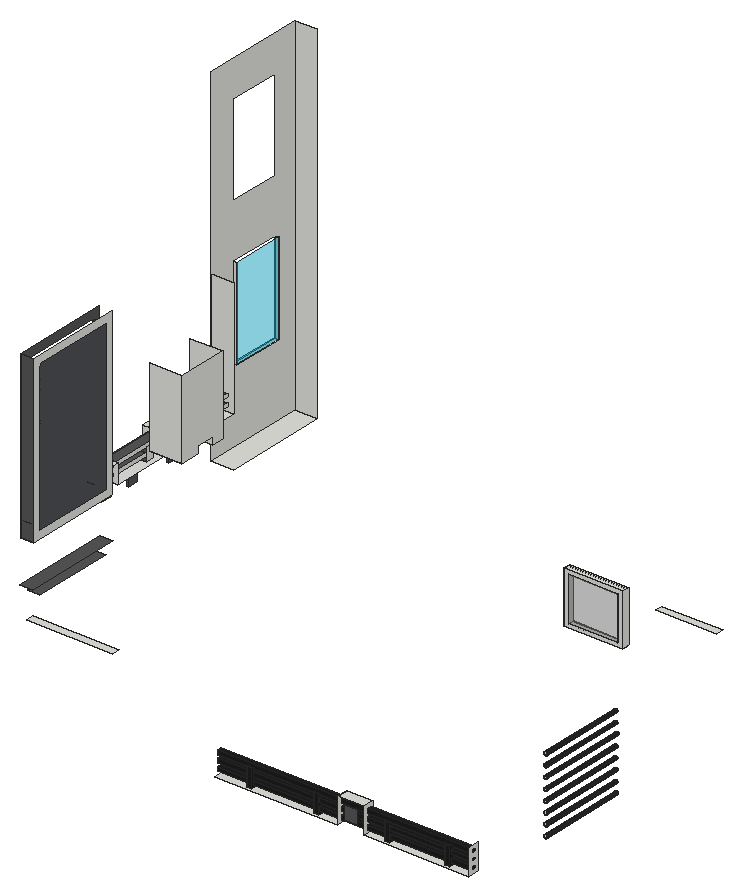
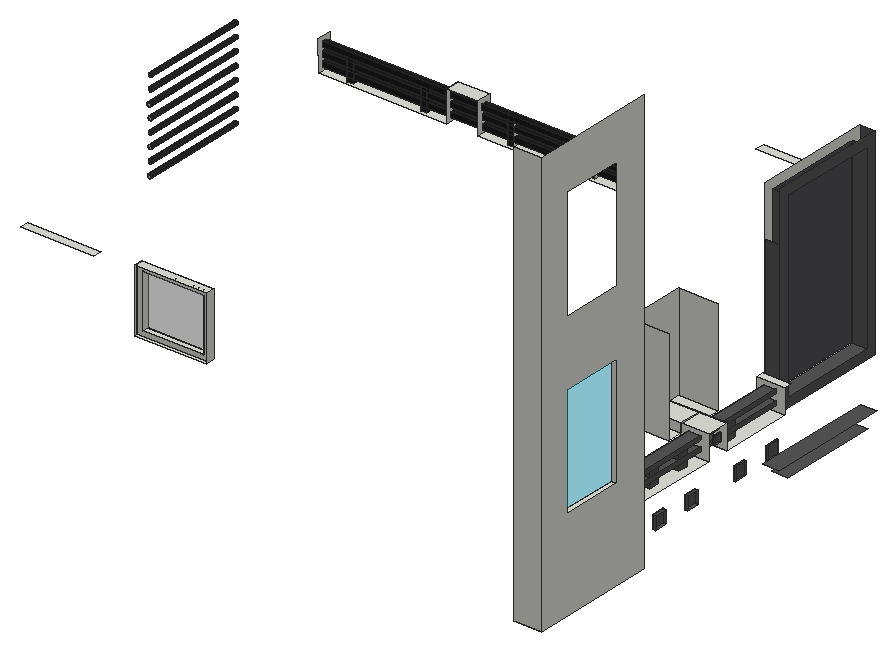
# SketchUp Ruby script. Lengths in inches.
U = 1.inch
M = Sketchup.active_model
def pt(a) = Geom::Point3d.new(a.map { |v| v * U })
def face(e, loops, mat)
  f = e.add_face(loops[0].map { |a| pt(a) })
  loops[1..].each { |l| e.add_face(l.map { |a| pt(a) }).erase! }
  f.material = f.back_material = mat if mat
  f
end
# faces: each face lists its corners as indices into pts; further lists are holes
def faces(e, pts, list, mat = nil) = list.each { |f| face(e, (f[0].is_a?(Array) ? f : [f]).map { |l| l.map { |i| pts[i] } }, mat) }
# xy, xz, yz: faces in a plane at the given z, y or x. An outline is a flat list of corners, or four numbers for a rectangle; further outlines are holes
def ring(l) = l.size == 4 ? [[l[0], l[1]], [l[2], l[1]], [l[2], l[3]], [l[0], l[3]]] : l.each_slice(2).to_a
def flat(e, list, mat, &to3) = list.each { |f| face(e, (f[0].is_a?(Array) ? f : [f]).map { |l| ring(l).map { |u, v| to3.(u, v) } }, mat) }
def xy(e, z, list, mat = nil) = flat(e, list, mat) { |x, y| [x, y, z] }
def xz(e, y, list, mat = nil) = flat(e, list, mat) { |x, z| [x, y, z] }
def yz(e, x, list, mat = nil) = flat(e, list, mat) { |y, z| [x, y, z] }
def lines(e, pts, list) = list.each { |a, b| e.add_line(pt(pts[a]), pt(pts[b])) }
# prism: a flat outline (further loops are holes) pulled along v
def prism(e, loops, v, mat = nil)
  f = face(e, loops, mat); d = Geom::Vector3d.new(v.map { |x| x * U })
  f.pushpull(f.normal.samedirection?(d) ? d.length : -d.length)
end
def box(e, o, s, mat = nil) = prism(e, [[o, [o[0] + s[0], o[1], o[2]], [o[0] + s[0], o[1] + s[1], o[2]], [o[0], o[1] + s[1], o[2]]]], [0, 0, s[2]], mat)
def at(x, y, z, deg = 0) = Geom::Transformation.translation(pt([x, y, z])) * Geom::Transformation.rotation(ORIGIN, Z_AXIS, deg.degrees)
def axes(o, x, y, z) = Geom::Transformation.new([*x, 0, *y, 0, *z, 0, *pt(o).to_a, 1])
def part(name) = M.definitions.add(name)
# library, detail: a bought-in or finely detailed component or shape, given as its bounding box
def library(name, o, s) = part(name).tap { |d| box(d.entities, o, s) }
def detail(e, o, s) = box(e.add_group.entities, o, s)
def put(e, d, t, mat = nil) = e.add_instance(d, t).tap { |i| i.material = mat if mat }
def group(e, t, mat = nil) = e.add_group.tap { |g| g.transformation = t; g.material = mat if mat }.entities
root = M.entities
M.materials.add("[Blinds Roman Hobbled Blue]").color = [81, 82, 87]
M.materials.add("[Color M06]").color = [86, 86, 86]
M.materials.add("[Color M08]").color = [30, 30, 30]
M.materials.add("[Translucent Glass Gray]").color = [128, 128, 128]
M.materials["[Translucent Glass Gray]"].alpha = 0.5
M.materials.add("[Translucent Glass Tinted]").color = [8, 201, 241]
M.materials["[Translucent Glass Tinted]"].alpha = 0.48
c1 = part("Group\#4")
xy(c1.entities,0,[[0,0,32.875,4]])
xy(c1.entities,2.47,[[2.47,0,30.4,4]])
xy(c1.entities,30.4,[[2.47,0,30.4,4]])
xy(c1.entities,32.875,[[0,0,32.875,4]])
xz(c1.entities,0,[[[0,0,32.875,32.875],[2.47,2.47,30.4,30.4]]])
xz(c1.entities,0,[[2.47,2.47,30.4,30.4]],"[Translucent Glass Gray]")
xz(c1.entities,4,[[[0,0,32.875,32.875],[2.47,2.47,30.4,30.4]]])
yz(c1.entities,0,[[0,0,4,32.875]])
yz(c1.entities,2.47,[[0,2.47,4,30.4]])
yz(c1.entities,30.4,[[0,2.47,4,30.4]])
yz(c1.entities,32.875,[[0,0,4,32.875]])
xy(root,185.33,[[67.1875,170.55,77.4375,235.42]],"[Color M06]")
xy(root,189.3125,[[[310.75,52.875,408.29,62.01],[387.07,55.5,391.07,59.5],[333.89,55.5,337.89,59.5]],[[428.93,52.875,512.75,62.01],[491.95,55.5,495.95,59.5],[443.64,55.5,447.64,59.5]]])
xy(root,190.375,[[59.3125,362.77,77.4375,446.27]])
xy(root,191.91,[[310.75,56.1,512.75,59.54]])
xy(root,192.66,[[67.1875,163.22,77.4375,242.75]],"[Color M06]")
xy(root,192.97,[[364.5,332.8125,411.32,338.8125]])
xy(root,195.34,[[310.75,56.1,512.75,59.54]],"[Color M08]")
xy(root,197.91,[[310.125,56.1,512.75,59.54]])
xy(root,201.34,[[310.125,56.1,512.75,59.54]],"[Color M08]")
xy(root,203.72,[[310.25,56.2,310.25,59.64,512.75,59.64,512.75,56.2,447.64,56.2,447.64,59.5,443.64,59.5,443.64,56.2],[443.64,56.2,447.64,59.5]])
xy(root,203.72,[[443.64,55.5,447.64,56.2]],"[Color M08]")
xy(root,204.125,[[333.89,55.5,337.89,59.5],[491.95,55.5,495.95,59.5]],"[Color M08]")
xy(root,204.5,[[387.07,55.5,391.07,59.5]],"[Color M08]")
xy(root,207.16,[[310.25,56.2,512.75,59.64]],"[Color M08]")
xy(root,208.79,[[59.3125,279.625,60.5,288.1875],[59.3125,318.6875,61.375,327.25],[59.3125,344.8125,61.3125,353.375]],"[Color M06]")
xy(root,209.47,[[59.3125,253.3125,60.3125,261.875]],"[Color M06]")
xy(root,209.8125,[[408.29,52.875,428.93,62.01]])
xy(root,217.35,[[59.3125,279.625,60.5,288.1875],[59.3125,318.6875,61.375,327.25],[59.3125,344.8125,61.3125,353.375]],"[Color M06]")
xy(root,218.03,[[59.3125,253.3125,60.3125,261.875]],"[Color M06]")
xy(root,225.6875,[[67.1875,164.28,77.4375,241.6875]],"[Color M06]")
xy(root,230,[[438.18,332.8125,486.18,338.8125]])
xy(root,231.95,[[67.1875,170.55,77.4375,235.42]],"[Color M06]")
xy(root,233.875,[[64.69,248.07,72.82,365.76]],"[Color M06]")
xy(root,234.22,[[364.5,332.8125,411.32,338.8125]])
xy(root,236.6875,[[64.69,248.07,72.82,365.76]],"[Color M06]")
xy(root,237.48,[[59.3125,300.15,60.1875,305.34]],"[Color M06]")
xy(root,240.34,[[77.4375,279.8125,103.125,294.97],[77.4375,309.77,103.125,319.875]])
xy(root,240.5,[[64.69,248.07,72.82,367.07]],"[Color M06]")
xy(root,242.66,[[59.3125,300.15,60.1875,305.34]],"[Color M06]")
xy(root,243.3125,[[64.69,248.07,72.82,367.07]],"[Color M06]")
xy(root,245.87,[[157.85,56.875,226.03,62.875]])
xy(root,246.02,[[59.3125,242.75,77.4375,248.07],[59.3125,294.97,77.4375,309.77],[77.4375,294.97,103.125,309.77]])
xy(root,250.33,[[59.3125,385.09,62.5,426.22]])
xz(root,52.875,[[414.09,194.96,423.78,205.53]],"[Color M06]")
xz(root,55.5,[[333.89,189.3125,337.89,204.125],[387.07,189.3125,391.07,204.5],[443.64,189.3125,447.64,203.72],[491.95,189.3125,495.95,204.125]],"[Color M08]")
xz(root,56.1,[[310.75,191.91,512.75,195.34],[310.125,197.91,512.75,201.34]],"[Color M08]")
xz(root,56.2,[[310.25,203.72,512.75,207.16]],"[Color M08]")
xz(root,59.5,[[333.89,189.3125,337.89,204.125],[387.07,189.3125,391.07,204.5],[443.64,189.3125,447.64,203.72],[491.95,189.3125,495.95,204.125]],"[Color M08]")
xz(root,59.54,[[310.75,191.91,512.75,195.34],[310.125,197.91,512.75,201.34]],"[Color M08]")
xz(root,59.64,[[310.25,203.72,512.75,207.16]],"[Color M08]")
xz(root,125.55,[[515.8,185.63,516.12,185.67,516.42,185.8,516.68,186,516.88,186.26,517.01,186.56,517.05,186.88,517.01,187.2,516.88,187.51,516.68,187.76,516.42,187.96,516.12,188.09,515.8,188.13,515.47,188.09,515.17,187.96,514.91,187.76,514.72,187.51,514.59,187.2,514.55,186.88,514.59,186.56,514.72,186.26,514.91,186,515.17,185.8,515.47,185.67],[515.8,194.07,516.12,194.11,516.42,194.24,516.68,194.43,516.88,194.69,517.01,194.99,517.05,195.32,517.01,195.64,516.88,195.94,516.68,196.2,516.42,196.4,516.12,196.53,515.8,196.57,515.47,196.53,515.17,196.4,514.91,196.2,514.72,195.94,514.59,195.64,514.55,195.32,514.59,194.99,514.72,194.69,514.91,194.43,515.17,194.24,515.47,194.11],[515.8,202.51,516.12,202.55,516.42,202.67,516.68,202.87,516.88,203.13,517.01,203.43,517.05,203.76,517.01,204.08,516.88,204.38,516.68,204.64,516.42,204.84,516.12,204.96,515.8,205.01,515.47,204.96,515.17,204.84,514.91,204.64,514.72,204.38,514.59,204.08,514.55,203.76,514.59,203.43,514.72,203.13,514.91,202.87,515.17,202.67,515.47,202.55],[515.8,210.94,516.12,210.99,516.42,211.11,516.68,211.31,516.88,211.57,517.01,211.87,517.05,212.19,517.01,212.52,516.88,212.82,516.68,213.08,516.42,213.28,516.12,213.4,515.8,213.44,515.47,213.4,515.17,213.28,514.91,213.08,514.72,212.82,514.59,212.52,514.55,212.19,514.59,211.87,514.72,211.57,514.91,211.31,515.17,211.11,515.47,210.99],[515.8,219.38,516.12,219.42,516.42,219.55,516.68,219.75,516.88,220.01,517.01,220.31,517.05,220.63,517.01,220.95,516.88,221.26,516.68,221.51,516.42,221.71,516.12,221.84,515.8,221.88,515.47,221.84,515.17,221.71,514.91,221.51,514.72,221.26,514.59,220.95,514.55,220.63,514.59,220.31,514.72,220.01,514.91,219.75,515.17,219.55,515.47,219.42],
  [515.8,227.82,516.12,227.86,516.42,227.99,516.68,228.18,516.88,228.44,517.01,228.74,517.05,229.07,517.01,229.39,516.88,229.69,516.68,229.95,516.42,230.15,516.12,230.28,515.8,230.32,515.47,230.28,515.17,230.15,514.91,229.95,514.72,229.69,514.59,229.39,514.55,229.07,514.59,228.74,514.72,228.44,514.91,228.18,515.17,227.99,515.47,227.86],[515.8,244.69,516.12,244.74,516.42,244.86,516.68,245.06,516.88,245.32,517.01,245.62,517.05,245.94,517.01,246.27,516.88,246.57,516.68,246.83,516.42,247.03,516.12,247.15,515.8,247.19,515.47,247.15,515.17,247.03,514.91,246.83,514.72,246.57,514.59,246.27,514.55,245.94,514.59,245.62,514.72,245.32,514.91,245.06,515.17,244.86,515.47,244.74]])
xz(root,164.28,[[67.1875,225.6875,77.4375,356.84]],"[Color M06]")
xz(root,170.55,[[67.1875,231.95,77.4375,350.58]],"[Color M06]")
xz(root,195.68,[[515.8,219.38,515.47,219.42,515.17,219.55,514.91,219.75,514.72,220.01,514.59,220.31,514.55,220.63,514.59,220.95,514.72,221.26,514.91,221.51,515.17,221.71,515.47,221.84,515.8,221.88,516.12,221.84,516.42,221.71,516.68,221.51,516.88,221.26,517.01,220.95,517.05,220.63,517.01,220.31,516.88,220.01,516.68,219.75,516.42,219.55,516.12,219.42]])
xz(root,195.74,[[515.8,202.51,515.47,202.55,515.17,202.67,514.91,202.87,514.72,203.13,514.59,203.43,514.55,203.76,514.59,204.08,514.72,204.38,514.91,204.64,515.17,204.84,515.47,204.96,515.8,205.01,516.12,204.96,516.42,204.84,516.68,204.64,516.88,204.38,517.01,204.08,517.05,203.76,517.01,203.43,516.88,203.13,516.68,202.87,516.42,202.67,516.12,202.55]])
xz(root,196.24,[[515.8,185.63,515.47,185.67,515.17,185.8,514.91,186,514.72,186.26,514.59,186.56,514.55,186.88,514.59,187.2,514.72,187.51,514.91,187.76,515.17,187.96,515.47,188.09,515.8,188.13,516.12,188.09,516.42,187.96,516.68,187.76,516.88,187.51,517.01,187.2,517.05,186.88,517.01,186.56,516.88,186.26,516.68,186,516.42,185.8,516.12,185.67]])
xz(root,196.68,[[515.8,227.82,515.47,227.86,515.17,227.99,514.91,228.18,514.72,228.44,514.59,228.74,514.55,229.07,514.59,229.39,514.72,229.69,514.91,229.95,515.17,230.15,515.47,230.28,515.8,230.32,516.12,230.28,516.42,230.15,516.68,229.95,516.88,229.69,517.01,229.39,517.05,229.07,517.01,228.74,516.88,228.44,516.68,228.18,516.42,227.99,516.12,227.86]])
xz(root,235.42,[[67.1875,231.95,77.4375,350.58]],"[Color M06]")
xz(root,241.6875,[[67.1875,225.6875,77.4375,323.97]],"[Color M06]")
xz(root,248.07,[[[59.3125,230.24,77.4375,246.02],[64.69,233.875,72.82,236.6875],[64.69,240.5,72.82,243.3125]],[64.69,233.875,72.82,236.6875],[64.69,240.5,72.82,243.3125]])
xz(root,253.3125,[[59.3125,209.47,60.3125,218.03]],"[Color M06]")
xz(root,261.875,[[59.3125,209.47,60.3125,218.03]],"[Color M06]")
xz(root,279.625,[[59.3125,208.79,60.5,217.35]],"[Color M06]")
xz(root,279.8125,[[77.4375,240.34,103.125,302.91]])
xz(root,288.1875,[[59.3125,208.79,60.5,217.35]],"[Color M06]")
xz(root,294.97,[[59.3125,229.95,77.4375,246.02],[77.4375,240.34,103.125,246.02]])
xz(root,300.15,[[59.3125,237.48,60.1875,242.66]],"[Color M06]")
xz(root,305.34,[[59.3125,237.48,60.1875,242.66]],"[Color M06]")
xz(root,309.77,[[59.3125,229.95,77.4375,246.02],[77.4375,240.34,103.125,246.02]])
xz(root,318.6875,[[59.3125,208.79,61.375,217.35]],"[Color M06]")
xz(root,319.875,[[77.4375,240.34,103.125,302.91]])
xz(root,327.25,[[59.3125,208.79,61.375,217.35]],"[Color M06]")
xz(root,344.8125,[[59.3125,208.79,61.3125,217.35]],"[Color M06]")
xz(root,353.375,[[59.3125,208.79,61.3125,217.35]],"[Color M06]")
xz(root,362.77,[[59.3125,230.24,77.4375,323.97]])
xz(root,365.76,[[64.69,233.875,72.82,236.6875]])
xz(root,367.07,[[64.69,240.5,72.82,243.3125]])
xz(root,385.09,[[59.3125,250.33,62.5,323.27]])
xz(root,426.22,[[59.3125,250.33,62.5,323.27]])
xz(root,446.27,[[59.3125,190.375,77.4375,468]])
yz(root,59.3125,[[[362.77,190.375,446.27,468],[385.09,365.83,426.22,438.77],[385.09,250.33,426.22,323.27]]])
yz(root,60.1875,[[300.15,237.48,305.34,242.66]],"[Color M06]")
yz(root,60.3125,[[253.3125,209.47,261.875,218.03]],"[Color M06]")
yz(root,60.5,[[279.625,208.79,288.1875,217.35]],"[Color M06]")
yz(root,61.3125,[[344.8125,208.79,353.375,217.35]],"[Color M06]")
yz(root,61.375,[[318.6875,208.79,327.25,217.35]],"[Color M06]")
yz(root,62.5,[[385.09,250.33,426.22,323.27]],"[Translucent Glass Tinted]")
yz(root,64.69,[[248.07,233.875,365.76,236.6875],[248.07,240.5,367.07,243.3125]],"[Color M06]")
yz(root,64.87,[[281.6,230.14,281.54,241.27,287.67,241.3,287.73,230.17],[321.17,230.14,321.11,240.77,327.23,240.8,327.29,230.17],[344.73,230.14,344.67,240.5,350.8,240.54,350.85,230.17]],"[Color M06]")
yz(root,67.1875,[[[164.28,225.6875,241.6875,356.84],[170.55,231.95,235.42,350.58]]],"[Color M06]")
yz(root,72.82,[[248.07,233.875,365.76,236.6875],[248.07,240.5,367.07,243.3125]])
yz(root,73.43,[[281.6,230.14,287.73,230.17,287.67,241.3,281.54,241.27],[321.17,230.14,327.29,230.17,327.23,240.8,321.11,240.77],[344.73,230.14,350.85,230.17,350.8,240.54,344.67,240.5]])
yz(root,77.4375,[[[164.28,225.6875,241.6875,356.84],[170.55,231.95,235.42,350.58]],[294.97,240.34,309.77,246.02]])
yz(root,77.4375,[[170.55,231.95,235.42,350.58]],"[Blinds Roman Hobbled Blue]")
yz(root,103.125,[[279.8125,240.34,279.8125,302.91,319.875,302.91,319.875,240.34,309.77,240.34,309.77,246.02,294.97,246.02,294.97,240.34]])
yz(root,310.125,[[56.1,197.91,59.54,201.34]])
yz(root,310.25,[[56.2,203.72,59.64,207.16]])
yz(root,333.89,[[55.5,189.3125,59.5,204.125]])
yz(root,337.89,[[55.5,189.3125,59.5,204.125]],"[Color M08]")
yz(root,364.5,[[332.8125,192.97,338.8125,234.22]])
yz(root,387.07,[[55.5,189.3125,59.5,204.5]])
yz(root,391.07,[[55.5,189.3125,59.5,204.5]],"[Color M08]")
yz(root,408.29,[[52.875,189.3125,62.01,209.8125]])
yz(root,411.32,[[332.8125,192.97,338.8125,234.22]])
yz(root,428.93,[[52.875,189.3125,62.01,209.8125]])
yz(root,443.64,[[55.5,189.3125,59.5,203.72]],"[Color M08]")
yz(root,447.64,[[55.5,189.3125,59.5,203.72]],"[Color M08]")
yz(root,491.95,[[55.5,189.3125,59.5,204.125]],"[Color M08]")
yz(root,495.95,[[55.5,189.3125,59.5,204.125]],"[Color M08]")
yz(root,512.75,[[[52.875,189.3125,52.875,209.8125,62.375,209.8125,62.01,189.3125],[56.2,203.72,59.64,207.16],[56.1,197.91,59.54,201.34],[56.1,191.91,59.54,195.34]]])
p = [[515.8,125.55,185.63],[515.47,125.55,185.67],[515.47,196.24,185.67],[515.8,196.24,185.63],[516.12,125.55,185.67],[516.12,196.24,185.67],
  [515.17,125.55,185.8],[515.17,196.24,185.8],[516.42,125.55,185.8],[516.42,196.24,185.8],[514.91,125.55,186],[514.91,196.24,186],
  [516.68,125.55,186],[516.68,196.24,186],[514.72,125.55,186.26],[514.72,196.24,186.26],[516.88,125.55,186.26],[516.88,196.24,186.26],
  [514.59,125.55,186.56],[514.59,196.24,186.56],[517.01,125.55,186.56],[517.01,196.24,186.56],[514.55,125.55,186.88],[514.55,196.24,186.88],
  [517.05,125.55,186.88],[517.05,196.24,186.88],[514.59,125.55,187.2],[514.59,196.24,187.2],[517.01,125.55,187.2],[517.01,196.24,187.2],
  [514.72,125.55,187.51],[514.72,196.24,187.51],[516.88,125.55,187.51],[516.88,196.24,187.51],[514.91,125.55,187.76],[514.91,196.24,187.76],
  [516.68,125.55,187.76],[516.68,196.24,187.76],[515.17,125.55,187.96],[515.17,196.24,187.96],[516.42,125.55,187.96],[516.42,196.24,187.96],
  [515.47,125.55,188.09],[515.47,196.24,188.09],[516.12,125.55,188.09],[516.12,196.24,188.09],[515.8,125.55,188.13],[515.8,196.24,188.13],
  [515.47,125.55,194.11],[515.17,125.55,194.24],[515.17,195.62,194.24],[515.47,195.62,194.11],[515.8,125.55,194.07],[515.8,195.62,194.07],
  [516.12,125.55,194.11],[516.12,195.62,194.11],[516.42,125.55,194.24],[516.42,195.62,194.24],[514.91,125.55,194.43],[514.91,195.62,194.43],
  [516.68,125.55,194.43],[516.68,195.62,194.43],[514.72,125.55,194.69],[514.72,195.62,194.69],[516.88,125.55,194.69],[516.88,195.62,194.69],
  [514.59,125.55,194.99],[514.59,195.62,194.99],[517.01,125.55,194.99],[517.01,195.62,194.99],[514.55,125.55,195.32],[514.55,195.62,195.32],
  [517.05,125.55,195.32],[517.05,195.62,195.32],[514.59,125.55,195.64],[514.59,195.62,195.64],[517.01,125.55,195.64],[517.01,195.62,195.64],
  [514.72,125.55,195.94],[514.72,195.62,195.94],[516.88,125.55,195.94],[516.88,195.62,195.94],[514.91,125.55,196.2],[514.91,195.62,196.2],
  [516.68,125.55,196.2],[516.68,195.62,196.2],[515.17,125.55,196.4],[515.17,195.62,196.4],[516.42,125.55,196.4],[516.42,195.62,196.4],
  [515.47,125.55,196.53],[515.47,195.62,196.53],[516.12,125.55,196.53],[516.12,195.62,196.53],[515.8,125.55,196.57],[515.8,195.62,196.57],
  [515.47,125.55,202.55],[515.17,125.55,202.67],[515.17,195.74,202.67],[515.47,195.74,202.55],[515.8,125.55,202.51],[515.8,195.74,202.51],
  [516.12,125.55,202.55],[516.12,195.74,202.55],[516.42,125.55,202.67],[516.42,195.74,202.67],[514.91,125.55,202.87],[514.91,195.74,202.87],
  [516.68,125.55,202.87],[516.68,195.74,202.87],[514.72,125.55,203.13],[514.72,195.74,203.13],[516.88,125.55,203.13],[516.88,195.74,203.13],
  [514.59,125.55,203.43],[514.59,195.74,203.43],[517.01,125.55,203.43],[517.01,195.74,203.43],[514.55,125.55,203.76],[514.55,195.74,203.76],
  [517.05,125.55,203.76],[517.05,195.74,203.76],[514.59,125.55,204.08],[514.59,195.74,204.08],[517.01,125.55,204.08],[517.01,195.74,204.08],
  [514.72,125.55,204.38],[514.72,195.74,204.38],[516.88,125.55,204.38],[516.88,195.74,204.38],[514.91,125.55,204.64],[514.91,195.74,204.64],
  [516.68,125.55,204.64],[516.68,195.74,204.64],[515.17,125.55,204.84],[515.17,195.74,204.84],[516.42,125.55,204.84],[516.42,195.74,204.84],
  [515.47,125.55,204.96],[515.47,195.74,204.96],[516.12,125.55,204.96],[516.12,195.74,204.96],[515.8,125.55,205.01],[515.8,195.74,205.01],
  [515.8,125.55,210.94],[515.47,125.55,210.99],[515.47,195.62,210.99],[515.8,195.62,210.94],[516.12,125.55,210.99],[516.12,195.62,210.99],
  [515.17,125.55,211.11],[515.17,195.62,211.11],[516.42,125.55,211.11],[516.42,195.62,211.11],[514.91,125.55,211.31],[514.91,195.62,211.31],
  [516.68,125.55,211.31],[516.68,195.62,211.31],[514.72,125.55,211.57],[514.72,195.62,211.57],[516.88,125.55,211.57],[516.88,195.62,211.57],
  [514.59,125.55,211.87],[514.59,195.62,211.87],[517.01,125.55,211.87],[517.01,195.62,211.87],[514.55,125.55,212.19],[514.55,195.62,212.19],
  [517.05,125.55,212.19],[517.05,195.62,212.19],[514.59,125.55,212.52],[514.59,195.62,212.52],[517.01,125.55,212.52],[517.01,195.62,212.52],
  [514.72,125.55,212.82],[514.72,195.62,212.82],[516.88,125.55,212.82],[516.88,195.62,212.82],[514.91,125.55,213.08],[514.91,195.62,213.08],
  [516.68,125.55,213.08],[516.68,195.62,213.08],[515.17,125.55,213.28],[515.17,195.62,213.28],[516.42,125.55,213.28],[516.42,195.62,213.28],
  [515.47,125.55,213.4],[515.47,195.62,213.4],[516.12,125.55,213.4],[516.12,195.62,213.4],[515.8,125.55,213.44],[515.8,195.62,213.44],
  [515.47,125.55,219.42],[515.17,125.55,219.55],[515.17,195.68,219.55],[515.47,195.68,219.42],[515.8,125.55,219.38],[515.8,195.68,219.38],
  [516.12,125.55,219.42],[516.12,195.68,219.42],[516.42,125.55,219.55],[516.42,195.68,219.55],[514.91,125.55,219.75],[514.91,195.68,219.75],
  [516.68,125.55,219.75],[516.68,195.68,219.75],[514.72,125.55,220.01],[514.72,195.68,220.01],[516.88,125.55,220.01],[516.88,195.68,220.01],
  [514.59,125.55,220.31],[514.59,195.68,220.31],[517.01,125.55,220.31],[517.01,195.68,220.31],[514.55,125.55,220.63],[514.55,195.68,220.63],
  [517.05,125.55,220.63],[517.05,195.68,220.63],[514.59,125.55,220.95],[514.59,195.68,220.95],[517.01,125.55,220.95],[517.01,195.68,220.95],
  [514.72,125.55,221.26],[514.72,195.68,221.26],[516.88,125.55,221.26],[516.88,195.68,221.26],[514.91,125.55,221.51],[514.91,195.68,221.51],
  [516.68,125.55,221.51],[516.68,195.68,221.51],[515.17,125.55,221.71],[515.17,195.68,221.71],[516.42,125.55,221.71],[516.42,195.68,221.71],
  [515.47,125.55,221.84],[515.47,195.68,221.84],[516.12,125.55,221.84],[516.12,195.68,221.84],[515.8,125.55,221.88],[515.8,195.68,221.88],
  [515.8,125.55,227.82],[515.47,125.55,227.86],[515.47,196.68,227.86],[515.8,196.68,227.82],[516.12,125.55,227.86],[516.12,196.68,227.86],
  [515.17,125.55,227.99],[515.17,196.68,227.99],[516.42,125.55,227.99],[516.42,196.68,227.99],[514.91,125.55,228.18],[514.91,196.68,228.18],
  [516.68,125.55,228.18],[516.68,196.68,228.18],[514.72,125.55,228.44],[514.72,196.68,228.44],[516.88,125.55,228.44],[516.88,196.68,228.44],
  [514.59,125.55,228.74],[514.59,196.68,228.74],[517.01,125.55,228.74],[517.01,196.68,228.74],[514.55,125.55,229.07],[514.55,196.68,229.07],
  [517.05,125.55,229.07],[517.05,196.68,229.07],[514.59,125.55,229.39],[514.59,196.68,229.39],[517.01,125.55,229.39],[517.01,196.68,229.39],
  [514.72,125.55,229.69],[514.72,196.68,229.69],[516.88,125.55,229.69],[516.88,196.68,229.69],[514.91,125.55,229.95],[514.91,196.68,229.95],
  [516.68,125.55,229.95],[516.68,196.68,229.95],[515.17,125.55,230.15],[515.17,196.68,230.15],[516.42,125.55,230.15],[516.42,196.68,230.15],
  [77.4375,248.07,230.24],[77.4375,294.97,229.95],[59.3125,294.97,229.95],[59.3125,248.07,230.24],[59.3125,362.77,230.24],[59.3125,309.77,229.95],
  [77.4375,309.77,229.95],[77.4375,362.77,230.24],[73.43,344.73,230.14],[64.87,344.73,230.14],[64.87,350.85,230.17],[73.43,350.85,230.17],
  [64.87,281.6,230.14],[73.43,281.6,230.14],[73.43,281.54,241.27],[64.87,281.54,241.27],[64.87,287.73,230.17],[73.43,287.73,230.17],
  [64.87,321.17,230.14],[73.43,321.17,230.14],[73.43,321.11,240.77],[64.87,321.11,240.77],[64.87,327.29,230.17],[73.43,327.29,230.17],
  [73.43,344.67,240.5],[64.87,344.67,240.5],[515.47,125.55,230.28],[515.47,196.68,230.28],[516.12,125.55,230.28],[516.12,196.68,230.28],
  [64.87,287.67,241.3],[73.43,287.67,241.3],[64.87,327.23,240.8],[73.43,327.23,240.8],[64.87,350.8,240.54],[73.43,350.8,240.54],
  [515.8,125.55,230.32],[515.8,196.68,230.32],[515.47,125.55,236.3],[515.17,125.55,236.42],[515.17,195.62,236.42],[515.47,195.62,236.3],
  [515.8,125.55,236.26],[515.8,195.62,236.26],[516.12,125.55,236.3],[516.12,195.62,236.3],[516.42,125.55,236.42],[516.42,195.62,236.42],
  [514.91,125.55,236.62],[514.91,195.62,236.62],[516.68,125.55,236.62],[516.68,195.62,236.62],[514.72,125.55,236.88],[514.72,195.62,236.88],
  [516.88,125.55,236.88],[516.88,195.62,236.88],[514.59,125.55,237.18],[514.59,195.62,237.18],[517.01,125.55,237.18],[517.01,195.62,237.18],
  [514.55,125.55,237.51],[514.55,195.62,237.51],[517.05,125.55,237.51],[517.05,195.62,237.51],[514.59,125.55,237.83],[514.59,195.62,237.83],
  [517.01,125.55,237.83],[517.01,195.62,237.83],[514.72,125.55,238.13],[514.72,195.62,238.13],[516.88,125.55,238.13],[516.88,195.62,238.13],
  [514.91,125.55,238.39],[514.91,195.62,238.39],[516.68,125.55,238.39],[516.68,195.62,238.39],[515.17,125.55,238.59],[515.17,195.62,238.59],
  [516.42,125.55,238.59],[516.42,195.62,238.59],[515.47,125.55,238.71],[515.47,195.62,238.71],[516.12,125.55,238.71],[516.12,195.62,238.71],
  [515.8,125.55,238.76],[515.8,195.62,238.76],[515.47,125.55,244.74],[515.17,125.55,244.86],[515.17,195.62,244.86],[515.47,195.62,244.74],
  [515.8,125.55,244.69],[515.8,195.62,244.69],[516.12,125.55,244.74],[516.12,195.62,244.74],[516.42,125.55,244.86],[516.42,195.62,244.86],
  [514.91,125.55,245.06],[514.91,195.62,245.06],[516.68,125.55,245.06],[516.68,195.62,245.06],[514.72,125.55,245.32],[514.72,195.62,245.32],
  [516.88,125.55,245.32],[516.88,195.62,245.32],[514.59,125.55,245.62],[514.59,195.62,245.62],[517.01,125.55,245.62],[517.01,195.62,245.62],
  [514.55,125.55,245.94],[514.55,195.62,245.94],[517.05,125.55,245.94],[517.05,195.62,245.94],[514.59,125.55,246.27],[514.59,195.62,246.27],
  [517.01,125.55,246.27],[517.01,195.62,246.27],[514.72,125.55,246.57],[514.72,195.62,246.57],[516.88,125.55,246.57],[516.88,195.62,246.57],
  [514.91,125.55,246.83],[514.91,195.62,246.83],[516.68,125.55,246.83],[516.68,195.62,246.83],[515.17,125.55,247.03],[515.17,195.62,247.03],
  [516.42,125.55,247.03],[516.42,195.62,247.03],[515.47,125.55,247.15],[515.47,195.62,247.15],[516.12,125.55,247.15],[516.12,195.62,247.15],
  [515.8,125.55,247.19],[515.8,195.62,247.19],[77.4375,153.86,245.85],[83.4375,153.86,245.85],[77.4375,217.18,245.85],[83.4375,217.18,245.85]]
faces(root,p,[[0,1,2,3],[4,0,3,5],[1,6,7,2],[8,4,5,9],[6,10,11,7],[12,8,9,13],[10,14,15,11],[16,12,13,17],
  [14,18,19,15],[20,16,17,21],[18,22,23,19],[24,20,21,25],[22,26,27,23],[28,24,25,29],[26,30,31,27],[32,28,29,33],
  [30,34,35,31],[36,32,33,37],[34,38,39,35],[40,36,37,41],[38,42,43,39],[44,40,41,45],[42,46,47,43],[46,44,45,47],
  [48,49,50,51],[52,48,51,53],[54,52,53,55],[56,54,55,57],[49,58,59,50],[60,56,57,61],[58,62,63,59],[64,60,61,65],
  [62,66,67,63],[68,64,65,69],[66,70,71,67],[72,68,69,73],[70,74,75,71],[76,72,73,77],[74,78,79,75],[80,76,77,81],
  [78,82,83,79],[84,80,81,85],[82,86,87,83],[88,84,85,89],[86,90,91,87],[92,88,89,93],[90,94,95,91],[94,92,93,95],
  [96,97,98,99],[100,96,99,101],[102,100,101,103],[104,102,103,105],[97,106,107,98],[108,104,105,109],[106,110,111,107],[112,108,109,113],
  [110,114,115,111],[116,112,113,117],[114,118,119,115],[120,116,117,121],[118,122,123,119],[124,120,121,125],[122,126,127,123],[128,124,125,129],
  [126,130,131,127],[132,128,129,133],[130,134,135,131],[136,132,133,137],[134,138,139,135],[140,136,137,141],[138,142,143,139],[142,140,141,143],
  [144,145,146,147],[148,144,147,149],[145,150,151,146],[152,148,149,153],[150,154,155,151],[156,152,153,157],[154,158,159,155],[160,156,157,161],
  [158,162,163,159],[164,160,161,165],[162,166,167,163],[168,164,165,169],[166,170,171,167],[172,168,169,173],[170,174,175,171],[176,172,173,177],
  [174,178,179,175],[180,176,177,181],[178,182,183,179],[184,180,181,185],[182,186,187,183],[188,184,185,189],[186,190,191,187],[190,188,189,191],
  [192,193,194,195],[196,192,195,197],[198,196,197,199],[200,198,199,201],[193,202,203,194],[204,200,201,205],[202,206,207,203],[208,204,205,209],
  [206,210,211,207],[212,208,209,213],[210,214,215,211],[216,212,213,217],[214,218,219,215],[220,216,217,221],[218,222,223,219],[224,220,221,225],
  [222,226,227,223],[228,224,225,229],[226,230,231,227],[232,228,229,233],[230,234,235,231],[236,232,233,237],[234,238,239,235],[238,236,237,239],
  [240,241,242,243],[244,240,243,245],[241,246,247,242],[248,244,245,249],[246,250,251,247],[252,248,249,253],[250,254,255,251],[256,252,253,257],
  [254,258,259,255],[260,256,257,261],[258,262,263,259],[264,260,261,265],[262,266,267,263],[268,264,265,269],[266,270,271,267],[272,268,269,273],
  [270,274,275,271],[276,272,273,277],[274,278,279,275],[280,276,277,281],[278,308,309,279],[310,280,281,311],[308,318,319,309],[318,310,311,319],
  [320,321,322,323],[324,320,323,325],[326,324,325,327],[328,326,327,329],[321,330,331,322],[332,328,329,333],[330,334,335,331],[336,332,333,337],
  [334,338,339,335],[340,336,337,341],[338,342,343,339],[344,340,341,345],[342,346,347,343],[348,344,345,349],[346,350,351,347],[352,348,349,353],
  [350,354,355,351],[356,352,353,357],[354,358,359,355],[360,356,357,361],[358,362,363,359],[364,360,361,365],[362,366,367,363],[366,364,365,367],
  [368,369,370,371],[372,368,371,373],[374,372,373,375],[376,374,375,377],[369,378,379,370],[380,376,377,381],[378,382,383,379],[384,380,381,385],
  [382,386,387,383],[388,384,385,389],[386,390,391,387],[392,388,389,393],[390,394,395,391],[396,392,393,397],[394,398,399,395],[400,396,397,401],
  [398,402,403,399],[404,400,401,405],[402,406,407,403],[408,404,405,409],[406,410,411,407],[412,408,409,413],[410,414,415,411],[414,412,413,415]],"[Color M08]")
faces(root,p,[[282,283,284,285],[[286,287,288,289],[290,291,292,293]],[295,294,298,299],[301,300,304,305],[290,291,292,293],[307,306,317,316],[303,302,315,314],[297,296,313,312]])
faces(root,p,[[294,295,296,297],[300,301,302,303],[291,290,306,307],[299,298,312,313],[305,304,314,315],[293,292,316,317]],"[Color M06]")
lines(root,p,[[416,417],[418,419]])
put(root,c1,axes([364.63,332.8125,192.97],[1.42,0,0],[0,1,0],[0,0,1.25475]))
